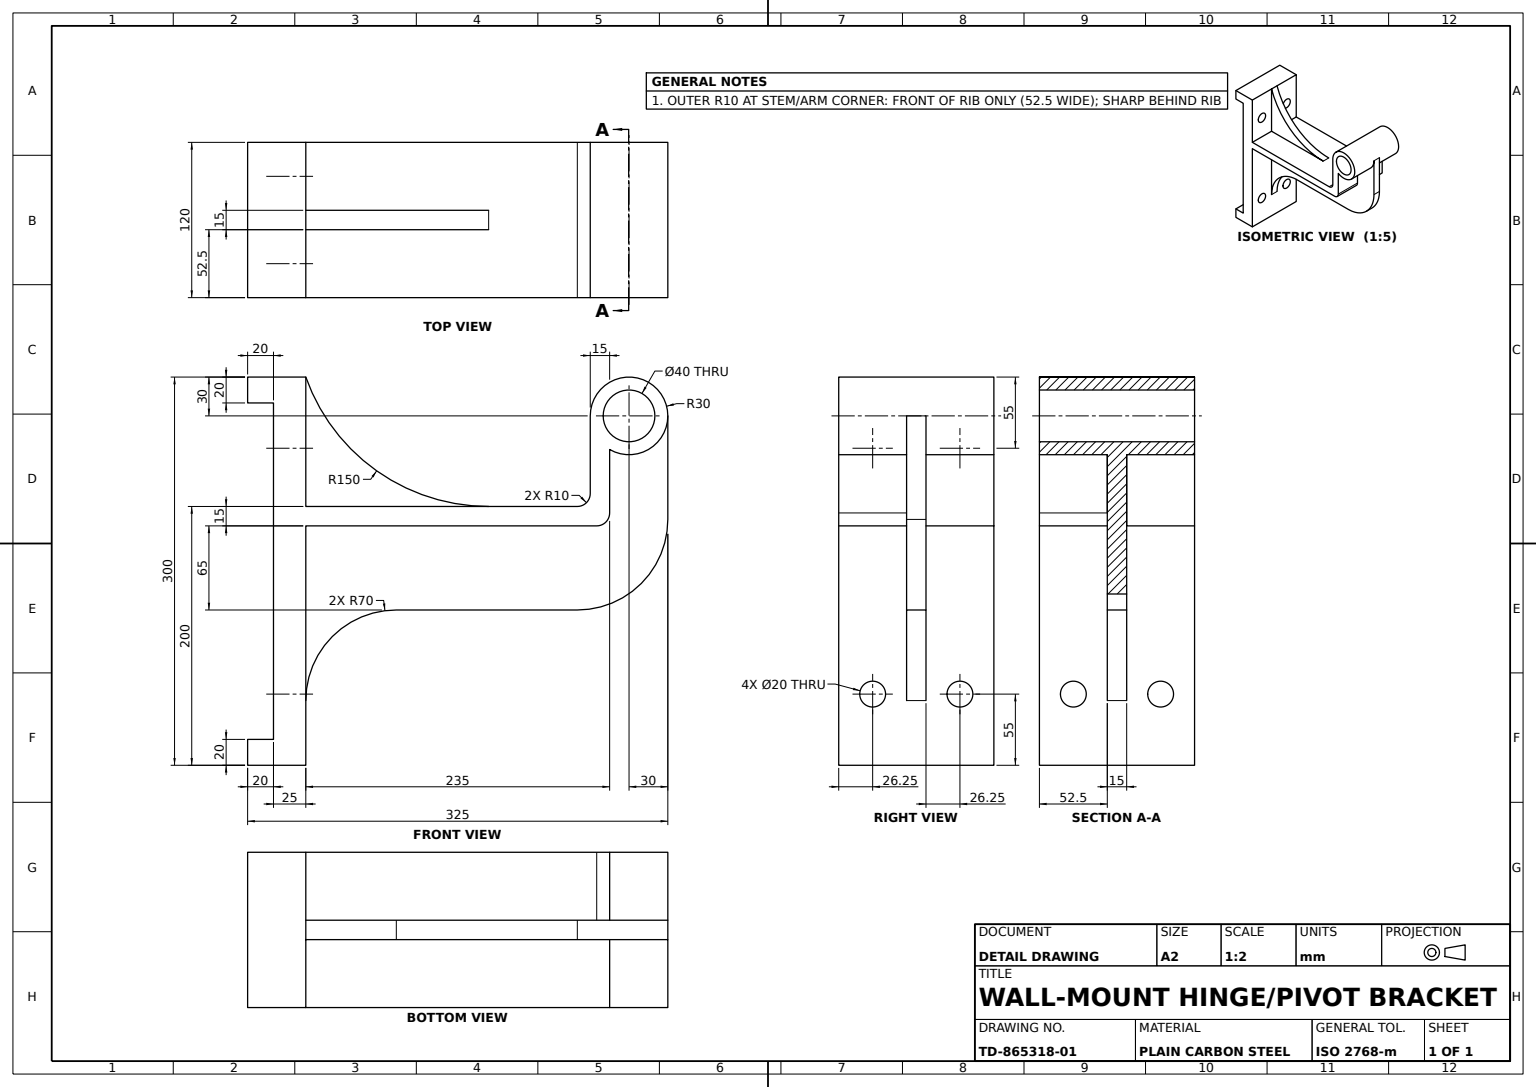
ISO-10303-21;
HEADER;
FILE_DESCRIPTION((''),'2;1');
FILE_NAME('','',(''),(''),'','','');
FILE_SCHEMA(('AUTOMOTIVE_DESIGN'));
ENDSEC;
DATA;
#1=APPLICATION_CONTEXT('');
#2=PRODUCT_CONTEXT('',#1,'mechanical');
#3=PRODUCT('','','',(#2));
#4=PRODUCT_DEFINITION_FORMATION('','',#3);
#5=PRODUCT_DEFINITION_CONTEXT('',#1,'design');
#6=PRODUCT_DEFINITION('','',#4,#5);
#7=PRODUCT_DEFINITION_SHAPE('','',#6);
#8=(LENGTH_UNIT()NAMED_UNIT(*)SI_UNIT(.MILLI.,.METRE.));
#9=(NAMED_UNIT(*)PLANE_ANGLE_UNIT()SI_UNIT($,.RADIAN.));
#10=(NAMED_UNIT(*)SI_UNIT($,.STERADIAN.)SOLID_ANGLE_UNIT());
#11=UNCERTAINTY_MEASURE_WITH_UNIT(LENGTH_MEASURE(1.E-05),#8,'distance_accuracy_value','');
#12=(GEOMETRIC_REPRESENTATION_CONTEXT(3)GLOBAL_UNCERTAINTY_ASSIGNED_CONTEXT((#11))GLOBAL_UNIT_ASSIGNED_CONTEXT((#8,#9,#10))REPRESENTATION_CONTEXT('',''));
#13=CARTESIAN_POINT('',(0.,120.,-292.5));
#14=VERTEX_POINT('',#13);
#15=CARTESIAN_POINT('',(0.,120.,-252.5));
#16=VERTEX_POINT('',#15);
#17=CARTESIAN_POINT('',(0.,120.,-272.5));
#18=DIRECTION('',(1.,0.,0.));
#19=DIRECTION('',(0.,0.,-1.));
#20=AXIS2_PLACEMENT_3D('',#17,#18,#19);
#21=CIRCLE('',#20,20.);
#22=EDGE_CURVE('',#14,#16,#21,.T.);
#23=ORIENTED_EDGE('',*,*,#22,.T.);
#24=CARTESIAN_POINT('',(-120.,120.,-252.5));
#25=VERTEX_POINT('',#24);
#26=VECTOR('',#18,1000.);
#27=LINE('',#24,#26);
#28=EDGE_CURVE('',#25,#16,#27,.T.);
#29=ORIENTED_EDGE('',*,*,#28,.F.);
#30=CARTESIAN_POINT('',(-120.,120.,-292.5));
#31=VERTEX_POINT('',#30);
#32=CARTESIAN_POINT('',(-120.,120.,-272.5));
#33=AXIS2_PLACEMENT_3D('',#32,#18,#19);
#34=CIRCLE('',#33,20.);
#35=EDGE_CURVE('',#31,#25,#34,.T.);
#36=ORIENTED_EDGE('',*,*,#35,.F.);
#37=LINE('',#30,#26);
#38=EDGE_CURVE('',#31,#14,#37,.T.);
#39=ORIENTED_EDGE('',*,*,#38,.T.);
#40=EDGE_LOOP('',(#23,#29,#36,#39));
#41=FACE_OUTER_BOUND('',#40,.T.);
#42=CYLINDRICAL_SURFACE('',#33,20.);
#43=ADVANCED_FACE('',(#41),#42,.F.);
#44=ORIENTED_EDGE('',*,*,#22,.F.);
#45=EDGE_CURVE('',#16,#14,#21,.T.);
#46=ORIENTED_EDGE('',*,*,#45,.F.);
#47=EDGE_LOOP('',(#44,#46));
#48=FACE_BOUND('',#47,.T.);
#49=CARTESIAN_POINT('',(0.,130.,22.5));
#50=VERTEX_POINT('',#49);
#51=CARTESIAN_POINT('',(0.,130.,2.5));
#52=VERTEX_POINT('',#51);
#53=VECTOR('',#19,1000.);
#54=LINE('',#49,#53);
#55=EDGE_CURVE('',#50,#52,#54,.T.);
#56=ORIENTED_EDGE('',*,*,#55,.T.);
#57=CARTESIAN_POINT('',(0.,-130.,2.5));
#58=VERTEX_POINT('',#57);
#59=DIRECTION('',(0.,-1.,0.));
#60=VECTOR('',#59,1000.);
#61=LINE('',#51,#60);
#62=EDGE_CURVE('',#52,#58,#61,.T.);
#63=ORIENTED_EDGE('',*,*,#62,.T.);
#64=CARTESIAN_POINT('',(0.,-130.,22.5));
#65=VERTEX_POINT('',#64);
#66=DIRECTION('',(0.,0.,1.));
#67=VECTOR('',#66,1000.);
#68=LINE('',#57,#67);
#69=EDGE_CURVE('',#58,#65,#68,.T.);
#70=ORIENTED_EDGE('',*,*,#69,.T.);
#71=CARTESIAN_POINT('',(0.,-150.,22.5));
#72=VERTEX_POINT('',#71);
#73=LINE('',#71,#60);
#74=EDGE_CURVE('',#65,#72,#73,.T.);
#75=ORIENTED_EDGE('',*,*,#74,.T.);
#76=CARTESIAN_POINT('',(0.,-150.,-22.5));
#77=VERTEX_POINT('',#76);
#78=LINE('',#71,#53);
#79=EDGE_CURVE('',#72,#77,#78,.T.);
#80=ORIENTED_EDGE('',*,*,#79,.T.);
#81=CARTESIAN_POINT('',(0.,35.,-22.5));
#82=VERTEX_POINT('',#81);
#83=DIRECTION('',(0.,1.,0.));
#84=VECTOR('',#83,1000.);
#85=LINE('',#76,#84);
#86=EDGE_CURVE('',#77,#82,#85,.T.);
#87=ORIENTED_EDGE('',*,*,#86,.T.);
#88=CARTESIAN_POINT('',(0.,35.,-247.5));
#89=VERTEX_POINT('',#88);
#90=CARTESIAN_POINT('',(0.,35.,-257.5));
#91=LINE('',#90,#67);
#92=EDGE_CURVE('',#89,#82,#91,.T.);
#93=ORIENTED_EDGE('',*,*,#92,.F.);
#94=CARTESIAN_POINT('',(0.,45.,-257.5));
#95=VERTEX_POINT('',#94);
#96=CARTESIAN_POINT('',(0.,45.,-247.5));
#97=AXIS2_PLACEMENT_3D('',#96,#18,#66);
#98=CIRCLE('',#97,10.);
#99=EDGE_CURVE('',#89,#95,#98,.T.);
#100=ORIENTED_EDGE('',*,*,#99,.T.);
#101=CARTESIAN_POINT('',(0.,94.019238,-257.5));
#102=VERTEX_POINT('',#101);
#103=CARTESIAN_POINT('',(0.,50.,-257.5));
#104=LINE('',#103,#60);
#105=EDGE_CURVE('',#102,#95,#104,.T.);
#106=ORIENTED_EDGE('',*,*,#105,.F.);
#107=CARTESIAN_POINT('',(0.,120.,-302.5));
#108=VERTEX_POINT('',#107);
#109=CIRCLE('',#20,30.);
#110=EDGE_CURVE('',#102,#108,#109,.T.);
#111=ORIENTED_EDGE('',*,*,#110,.T.);
#112=CARTESIAN_POINT('',(0.,120.,-242.5));
#113=VERTEX_POINT('',#112);
#114=EDGE_CURVE('',#108,#113,#109,.T.);
#115=ORIENTED_EDGE('',*,*,#114,.T.);
#116=CARTESIAN_POINT('',(0.,60.,-242.5));
#117=VERTEX_POINT('',#116);
#118=LINE('',#112,#60);
#119=EDGE_CURVE('',#113,#117,#118,.T.);
#120=ORIENTED_EDGE('',*,*,#119,.T.);
#121=CARTESIAN_POINT('',(0.,50.,-232.5));
#122=VERTEX_POINT('',#121);
#123=CARTESIAN_POINT('',(0.,60.,-232.5));
#124=DIRECTION('',(-1.,0.,0.));
#125=AXIS2_PLACEMENT_3D('',#123,#124,#66);
#126=CIRCLE('',#125,10.);
#127=EDGE_CURVE('',#117,#122,#126,.T.);
#128=ORIENTED_EDGE('',*,*,#127,.T.);
#129=CARTESIAN_POINT('',(0.,50.,-22.5));
#130=VERTEX_POINT('',#129);
#131=LINE('',#103,#67);
#132=EDGE_CURVE('',#122,#130,#131,.T.);
#133=ORIENTED_EDGE('',*,*,#132,.T.);
#134=CARTESIAN_POINT('',(0.,150.,-22.5));
#135=VERTEX_POINT('',#134);
#136=EDGE_CURVE('',#130,#135,#85,.T.);
#137=ORIENTED_EDGE('',*,*,#136,.T.);
#138=CARTESIAN_POINT('',(0.,150.,22.5));
#139=VERTEX_POINT('',#138);
#140=LINE('',#138,#67);
#141=EDGE_CURVE('',#135,#139,#140,.T.);
#142=ORIENTED_EDGE('',*,*,#141,.T.);
#143=LINE('',#49,#60);
#144=EDGE_CURVE('',#139,#50,#143,.T.);
#145=ORIENTED_EDGE('',*,*,#144,.T.);
#146=EDGE_LOOP('',(#56,#63,#70,#75,#80,#87,#93,#100,#106,#111,#115,#120,#128,#133,#137,#142,#145));
#147=FACE_OUTER_BOUND('',#146,.T.);
#148=CARTESIAN_POINT('',(0.,0.,0.));
#149=AXIS2_PLACEMENT_3D('',#148,#124,#66);
#150=PLANE('',#149);
#151=ADVANCED_FACE('',(#48,#147),#150,.F.);
#152=CARTESIAN_POINT('',(-67.5,150.,-22.5));
#153=VERTEX_POINT('',#152);
#154=CARTESIAN_POINT('',(-52.5,150.,-22.5));
#155=VERTEX_POINT('',#154);
#156=CARTESIAN_POINT('',(-60.,150.,-22.5));
#157=LINE('',#156,#26);
#158=EDGE_CURVE('',#153,#155,#157,.T.);
#159=ORIENTED_EDGE('',*,*,#158,.F.);
#160=CARTESIAN_POINT('',(-120.,150.,-22.5));
#161=VERTEX_POINT('',#160);
#162=LINE('',#160,#26);
#163=EDGE_CURVE('',#161,#153,#162,.T.);
#164=ORIENTED_EDGE('',*,*,#163,.F.);
#165=CARTESIAN_POINT('',(-120.,150.,22.5));
#166=VERTEX_POINT('',#165);
#167=LINE('',#165,#67);
#168=EDGE_CURVE('',#161,#166,#167,.T.);
#169=ORIENTED_EDGE('',*,*,#168,.T.);
#170=LINE('',#165,#26);
#171=EDGE_CURVE('',#166,#139,#170,.T.);
#172=ORIENTED_EDGE('',*,*,#171,.T.);
#173=ORIENTED_EDGE('',*,*,#141,.F.);
#174=EDGE_CURVE('',#155,#135,#162,.T.);
#175=ORIENTED_EDGE('',*,*,#174,.F.);
#176=EDGE_LOOP('',(#159,#164,#169,#172,#173,#175));
#177=FACE_OUTER_BOUND('',#176,.T.);
#178=AXIS2_PLACEMENT_3D('',#165,#83,#66);
#179=PLANE('',#178);
#180=ADVANCED_FACE('',(#177),#179,.T.);
#181=CARTESIAN_POINT('',(-67.5,-30.,-92.5));
#182=VERTEX_POINT('',#181);
#183=CARTESIAN_POINT('',(-67.5,-30.,-232.5));
#184=VERTEX_POINT('',#183);
#185=LINE('',#181,#53);
#186=EDGE_CURVE('',#182,#184,#185,.T.);
#187=ORIENTED_EDGE('',*,*,#186,.F.);
#188=CARTESIAN_POINT('',(-67.5,-100.,-22.5));
#189=VERTEX_POINT('',#188);
#190=CARTESIAN_POINT('',(-67.5,-100.,-92.5));
#191=AXIS2_PLACEMENT_3D('',#190,#124,#66);
#192=CIRCLE('',#191,70.);
#193=EDGE_CURVE('',#189,#182,#192,.T.);
#194=ORIENTED_EDGE('',*,*,#193,.F.);
#195=CARTESIAN_POINT('',(-67.5,35.,-22.5));
#196=VERTEX_POINT('',#195);
#197=LINE('',#188,#60);
#198=EDGE_CURVE('',#196,#189,#197,.T.);
#199=ORIENTED_EDGE('',*,*,#198,.F.);
#200=CARTESIAN_POINT('',(-67.5,35.,-257.5));
#201=VERTEX_POINT('',#200);
#202=LINE('',#195,#67);
#203=EDGE_CURVE('',#201,#196,#202,.T.);
#204=ORIENTED_EDGE('',*,*,#203,.F.);
#205=CARTESIAN_POINT('',(-67.5,94.019238,-257.5));
#206=VERTEX_POINT('',#205);
#207=LINE('',#200,#60);
#208=EDGE_CURVE('',#206,#201,#207,.T.);
#209=ORIENTED_EDGE('',*,*,#208,.F.);
#210=CARTESIAN_POINT('',(-67.5,120.,-302.5));
#211=VERTEX_POINT('',#210);
#212=CARTESIAN_POINT('',(-67.5,120.,-272.5));
#213=AXIS2_PLACEMENT_3D('',#212,#124,#19);
#214=CIRCLE('',#213,30.);
#215=EDGE_CURVE('',#211,#206,#214,.T.);
#216=ORIENTED_EDGE('',*,*,#215,.F.);
#217=CARTESIAN_POINT('',(-67.5,40.,-302.5));
#218=VERTEX_POINT('',#217);
#219=LINE('',#210,#84);
#220=EDGE_CURVE('',#218,#211,#219,.T.);
#221=ORIENTED_EDGE('',*,*,#220,.F.);
#222=CARTESIAN_POINT('',(-67.5,40.,-232.5));
#223=AXIS2_PLACEMENT_3D('',#222,#18,#19);
#224=CIRCLE('',#223,70.);
#225=EDGE_CURVE('',#184,#218,#224,.T.);
#226=ORIENTED_EDGE('',*,*,#225,.F.);
#227=EDGE_LOOP('',(#187,#194,#199,#204,#209,#216,#221,#226));
#228=FACE_OUTER_BOUND('',#227,.T.);
#229=AXIS2_PLACEMENT_3D('',#212,#18,#19);
#230=PLANE('',#229);
#231=ADVANCED_FACE('',(#228),#230,.F.);
#232=CARTESIAN_POINT('',(-120.,-130.,2.5));
#233=VERTEX_POINT('',#232);
#234=CARTESIAN_POINT('',(-120.,-130.,22.5));
#235=VERTEX_POINT('',#234);
#236=LINE('',#232,#67);
#237=EDGE_CURVE('',#233,#235,#236,.T.);
#238=ORIENTED_EDGE('',*,*,#237,.T.);
#239=LINE('',#234,#26);
#240=EDGE_CURVE('',#235,#65,#239,.T.);
#241=ORIENTED_EDGE('',*,*,#240,.T.);
#242=ORIENTED_EDGE('',*,*,#69,.F.);
#243=LINE('',#232,#26);
#244=EDGE_CURVE('',#233,#58,#243,.T.);
#245=ORIENTED_EDGE('',*,*,#244,.F.);
#246=EDGE_LOOP('',(#238,#241,#242,#245));
#247=FACE_OUTER_BOUND('',#246,.T.);
#248=AXIS2_PLACEMENT_3D('',#232,#83,#66);
#249=PLANE('',#248);
#250=ADVANCED_FACE('',(#247),#249,.T.);
#251=CARTESIAN_POINT('',(-120.,-150.,22.5));
#252=VERTEX_POINT('',#251);
#253=CARTESIAN_POINT('',(-120.,-150.,-22.5));
#254=VERTEX_POINT('',#253);
#255=LINE('',#251,#53);
#256=EDGE_CURVE('',#252,#254,#255,.T.);
#257=ORIENTED_EDGE('',*,*,#256,.F.);
#258=LINE('',#251,#60);
#259=EDGE_CURVE('',#235,#252,#258,.T.);
#260=ORIENTED_EDGE('',*,*,#259,.F.);
#261=ORIENTED_EDGE('',*,*,#237,.F.);
#262=CARTESIAN_POINT('',(-120.,130.,2.5));
#263=VERTEX_POINT('',#262);
#264=LINE('',#262,#60);
#265=EDGE_CURVE('',#263,#233,#264,.T.);
#266=ORIENTED_EDGE('',*,*,#265,.F.);
#267=CARTESIAN_POINT('',(-120.,130.,22.5));
#268=VERTEX_POINT('',#267);
#269=LINE('',#267,#53);
#270=EDGE_CURVE('',#268,#263,#269,.T.);
#271=ORIENTED_EDGE('',*,*,#270,.F.);
#272=LINE('',#267,#60);
#273=EDGE_CURVE('',#166,#268,#272,.T.);
#274=ORIENTED_EDGE('',*,*,#273,.F.);
#275=ORIENTED_EDGE('',*,*,#168,.F.);
#276=CARTESIAN_POINT('',(-120.,50.,-22.5));
#277=VERTEX_POINT('',#276);
#278=LINE('',#253,#84);
#279=EDGE_CURVE('',#277,#161,#278,.T.);
#280=ORIENTED_EDGE('',*,*,#279,.F.);
#281=CARTESIAN_POINT('',(-120.,50.,-232.5));
#282=VERTEX_POINT('',#281);
#283=CARTESIAN_POINT('',(-120.,50.,-257.5));
#284=LINE('',#283,#67);
#285=EDGE_CURVE('',#282,#277,#284,.T.);
#286=ORIENTED_EDGE('',*,*,#285,.F.);
#287=CARTESIAN_POINT('',(-120.,60.,-242.5));
#288=VERTEX_POINT('',#287);
#289=CARTESIAN_POINT('',(-120.,60.,-232.5));
#290=AXIS2_PLACEMENT_3D('',#289,#18,#66);
#291=CIRCLE('',#290,10.);
#292=EDGE_CURVE('',#282,#288,#291,.T.);
#293=ORIENTED_EDGE('',*,*,#292,.T.);
#294=CARTESIAN_POINT('',(-120.,120.,-242.5));
#295=VERTEX_POINT('',#294);
#296=LINE('',#294,#60);
#297=EDGE_CURVE('',#295,#288,#296,.T.);
#298=ORIENTED_EDGE('',*,*,#297,.F.);
#299=CARTESIAN_POINT('',(-120.,120.,-302.5));
#300=VERTEX_POINT('',#299);
#301=CIRCLE('',#33,30.);
#302=EDGE_CURVE('',#300,#295,#301,.T.);
#303=ORIENTED_EDGE('',*,*,#302,.F.);
#304=CARTESIAN_POINT('',(-120.,94.019238,-257.5));
#305=VERTEX_POINT('',#304);
#306=EDGE_CURVE('',#305,#300,#301,.T.);
#307=ORIENTED_EDGE('',*,*,#306,.F.);
#308=CARTESIAN_POINT('',(-120.,35.,-257.5));
#309=VERTEX_POINT('',#308);
#310=LINE('',#283,#84);
#311=EDGE_CURVE('',#309,#305,#310,.T.);
#312=ORIENTED_EDGE('',*,*,#311,.F.);
#313=CARTESIAN_POINT('',(-120.,35.,-22.5));
#314=VERTEX_POINT('',#313);
#315=LINE('',#308,#67);
#316=EDGE_CURVE('',#309,#314,#315,.T.);
#317=ORIENTED_EDGE('',*,*,#316,.T.);
#318=EDGE_CURVE('',#254,#314,#278,.T.);
#319=ORIENTED_EDGE('',*,*,#318,.F.);
#320=EDGE_LOOP('',(#257,#260,#261,#266,#271,#274,#275,#280,#286,#293,#298,#303,#307,#312,#317,#319));
#321=FACE_OUTER_BOUND('',#320,.T.);
#322=ORIENTED_EDGE('',*,*,#35,.T.);
#323=EDGE_CURVE('',#25,#31,#34,.T.);
#324=ORIENTED_EDGE('',*,*,#323,.T.);
#325=EDGE_LOOP('',(#322,#324));
#326=FACE_BOUND('',#325,.T.);
#327=CARTESIAN_POINT('',(-120.,0.,0.));
#328=AXIS2_PLACEMENT_3D('',#327,#124,#66);
#329=PLANE('',#328);
#330=ADVANCED_FACE('',(#321,#326),#329,.T.);
#331=CARTESIAN_POINT('',(-103.75,95.,2.5));
#332=VERTEX_POINT('',#331);
#333=CARTESIAN_POINT('',(-103.75,95.,-22.5));
#334=VERTEX_POINT('',#333);
#335=CARTESIAN_POINT('',(-103.75,95.,22.5));
#336=LINE('',#335,#53);
#337=EDGE_CURVE('',#332,#334,#336,.T.);
#338=ORIENTED_EDGE('',*,*,#337,.F.);
#339=CARTESIAN_POINT('',(-83.75,95.,2.5));
#340=VERTEX_POINT('',#339);
#341=CARTESIAN_POINT('',(-93.75,95.,2.5));
#342=AXIS2_PLACEMENT_3D('',#341,#66,#59);
#343=CIRCLE('',#342,10.);
#344=EDGE_CURVE('',#332,#340,#343,.T.);
#345=ORIENTED_EDGE('',*,*,#344,.T.);
#346=CARTESIAN_POINT('',(-83.75,95.,-22.5));
#347=VERTEX_POINT('',#346);
#348=CARTESIAN_POINT('',(-83.75,95.,22.5));
#349=LINE('',#348,#53);
#350=EDGE_CURVE('',#340,#347,#349,.T.);
#351=ORIENTED_EDGE('',*,*,#350,.T.);
#352=CARTESIAN_POINT('',(-93.75,95.,-22.5));
#353=AXIS2_PLACEMENT_3D('',#352,#19,#124);
#354=CIRCLE('',#353,10.);
#355=EDGE_CURVE('',#347,#334,#354,.T.);
#356=ORIENTED_EDGE('',*,*,#355,.T.);
#357=EDGE_LOOP('',(#338,#345,#351,#356));
#358=FACE_OUTER_BOUND('',#357,.T.);
#359=CARTESIAN_POINT('',(-93.75,95.,22.5));
#360=AXIS2_PLACEMENT_3D('',#359,#19,#124);
#361=CYLINDRICAL_SURFACE('',#360,10.);
#362=ADVANCED_FACE('',(#358),#361,.F.);
#363=CARTESIAN_POINT('',(-52.5,50.,-163.921356));
#364=VERTEX_POINT('',#363);
#365=CARTESIAN_POINT('',(-52.5,200.,-163.921356));
#366=AXIS2_PLACEMENT_3D('',#365,#18,#19);
#367=CIRCLE('',#366,150.);
#368=EDGE_CURVE('',#155,#364,#367,.T.);
#369=ORIENTED_EDGE('',*,*,#368,.T.);
#370=CARTESIAN_POINT('',(-67.5,50.,-163.921356));
#371=VERTEX_POINT('',#370);
#372=CARTESIAN_POINT('',(-60.,50.,-163.921356));
#373=LINE('',#372,#26);
#374=EDGE_CURVE('',#371,#364,#373,.T.);
#375=ORIENTED_EDGE('',*,*,#374,.F.);
#376=CARTESIAN_POINT('',(-67.5,200.,-163.921356));
#377=AXIS2_PLACEMENT_3D('',#376,#18,#19);
#378=CIRCLE('',#377,150.);
#379=EDGE_CURVE('',#153,#371,#378,.T.);
#380=ORIENTED_EDGE('',*,*,#379,.F.);
#381=ORIENTED_EDGE('',*,*,#158,.T.);
#382=EDGE_LOOP('',(#369,#375,#380,#381));
#383=FACE_OUTER_BOUND('',#382,.T.);
#384=CARTESIAN_POINT('',(-60.,200.,-163.921356));
#385=AXIS2_PLACEMENT_3D('',#384,#18,#19);
#386=CYLINDRICAL_SURFACE('',#385,150.);
#387=ADVANCED_FACE('',(#383),#386,.F.);
#388=CARTESIAN_POINT('',(-36.25,95.,2.5));
#389=VERTEX_POINT('',#388);
#390=CARTESIAN_POINT('',(-16.25,95.,2.5));
#391=VERTEX_POINT('',#390);
#392=CARTESIAN_POINT('',(-26.25,95.,2.5));
#393=AXIS2_PLACEMENT_3D('',#392,#66,#59);
#394=CIRCLE('',#393,10.);
#395=EDGE_CURVE('',#389,#391,#394,.T.);
#396=ORIENTED_EDGE('',*,*,#395,.T.);
#397=CARTESIAN_POINT('',(-16.25,95.,-22.5));
#398=VERTEX_POINT('',#397);
#399=CARTESIAN_POINT('',(-16.25,95.,22.5));
#400=LINE('',#399,#53);
#401=EDGE_CURVE('',#391,#398,#400,.T.);
#402=ORIENTED_EDGE('',*,*,#401,.T.);
#403=CARTESIAN_POINT('',(-36.25,95.,-22.5));
#404=VERTEX_POINT('',#403);
#405=CARTESIAN_POINT('',(-26.25,95.,-22.5));
#406=AXIS2_PLACEMENT_3D('',#405,#19,#124);
#407=CIRCLE('',#406,10.);
#408=EDGE_CURVE('',#398,#404,#407,.T.);
#409=ORIENTED_EDGE('',*,*,#408,.T.);
#410=CARTESIAN_POINT('',(-36.25,95.,22.5));
#411=LINE('',#410,#53);
#412=EDGE_CURVE('',#389,#404,#411,.T.);
#413=ORIENTED_EDGE('',*,*,#412,.F.);
#414=EDGE_LOOP('',(#396,#402,#409,#413));
#415=FACE_OUTER_BOUND('',#414,.T.);
#416=CARTESIAN_POINT('',(-26.25,95.,22.5));
#417=AXIS2_PLACEMENT_3D('',#416,#19,#124);
#418=CYLINDRICAL_SURFACE('',#417,10.);
#419=ADVANCED_FACE('',(#415),#418,.F.);
#420=CARTESIAN_POINT('',(-52.5,50.,-22.5));
#421=VERTEX_POINT('',#420);
#422=CARTESIAN_POINT('',(-52.5,50.,-257.5));
#423=LINE('',#422,#67);
#424=EDGE_CURVE('',#364,#421,#423,.T.);
#425=ORIENTED_EDGE('',*,*,#424,.F.);
#426=ORIENTED_EDGE('',*,*,#368,.F.);
#427=CARTESIAN_POINT('',(-52.5,-150.,-22.5));
#428=LINE('',#427,#60);
#429=EDGE_CURVE('',#155,#421,#428,.T.);
#430=ORIENTED_EDGE('',*,*,#429,.T.);
#431=EDGE_LOOP('',(#425,#426,#430));
#432=FACE_OUTER_BOUND('',#431,.T.);
#433=CARTESIAN_POINT('',(-52.5,0.,-140.));
#434=AXIS2_PLACEMENT_3D('',#433,#18,#19);
#435=PLANE('',#434);
#436=ADVANCED_FACE('',(#432),#435,.T.);
#437=ORIENTED_EDGE('',*,*,#429,.F.);
#438=ORIENTED_EDGE('',*,*,#174,.T.);
#439=ORIENTED_EDGE('',*,*,#136,.F.);
#440=LINE('',#129,#26);
#441=EDGE_CURVE('',#421,#130,#440,.T.);
#442=ORIENTED_EDGE('',*,*,#441,.F.);
#443=EDGE_LOOP('',(#437,#438,#439,#442));
#444=FACE_OUTER_BOUND('',#443,.T.);
#445=ORIENTED_EDGE('',*,*,#408,.F.);
#446=EDGE_CURVE('',#404,#398,#407,.T.);
#447=ORIENTED_EDGE('',*,*,#446,.F.);
#448=EDGE_LOOP('',(#445,#447));
#449=FACE_BOUND('',#448,.T.);
#450=AXIS2_PLACEMENT_3D('',#253,#19,#124);
#451=PLANE('',#450);
#452=ADVANCED_FACE('',(#444,#449),#451,.T.);
#453=ORIENTED_EDGE('',*,*,#401,.F.);
#454=EDGE_CURVE('',#391,#389,#394,.T.);
#455=ORIENTED_EDGE('',*,*,#454,.T.);
#456=ORIENTED_EDGE('',*,*,#412,.T.);
#457=ORIENTED_EDGE('',*,*,#446,.T.);
#458=EDGE_LOOP('',(#453,#455,#456,#457));
#459=FACE_OUTER_BOUND('',#458,.T.);
#460=ADVANCED_FACE('',(#459),#418,.F.);
#461=CARTESIAN_POINT('',(-16.25,-95.,2.5));
#462=VERTEX_POINT('',#461);
#463=CARTESIAN_POINT('',(-16.25,-95.,-22.5));
#464=VERTEX_POINT('',#463);
#465=CARTESIAN_POINT('',(-16.25,-95.,22.5));
#466=LINE('',#465,#53);
#467=EDGE_CURVE('',#462,#464,#466,.T.);
#468=ORIENTED_EDGE('',*,*,#467,.T.);
#469=CARTESIAN_POINT('',(-36.25,-95.,-22.5));
#470=VERTEX_POINT('',#469);
#471=CARTESIAN_POINT('',(-26.25,-95.,-22.5));
#472=AXIS2_PLACEMENT_3D('',#471,#19,#124);
#473=CIRCLE('',#472,10.);
#474=EDGE_CURVE('',#464,#470,#473,.T.);
#475=ORIENTED_EDGE('',*,*,#474,.T.);
#476=CARTESIAN_POINT('',(-36.25,-95.,2.5));
#477=VERTEX_POINT('',#476);
#478=CARTESIAN_POINT('',(-36.25,-95.,22.5));
#479=LINE('',#478,#53);
#480=EDGE_CURVE('',#477,#470,#479,.T.);
#481=ORIENTED_EDGE('',*,*,#480,.F.);
#482=CARTESIAN_POINT('',(-26.25,-95.,2.5));
#483=AXIS2_PLACEMENT_3D('',#482,#66,#59);
#484=CIRCLE('',#483,10.);
#485=EDGE_CURVE('',#477,#462,#484,.T.);
#486=ORIENTED_EDGE('',*,*,#485,.T.);
#487=EDGE_LOOP('',(#468,#475,#481,#486));
#488=FACE_OUTER_BOUND('',#487,.T.);
#489=CARTESIAN_POINT('',(-26.25,-95.,22.5));
#490=AXIS2_PLACEMENT_3D('',#489,#19,#124);
#491=CYLINDRICAL_SURFACE('',#490,10.);
#492=ADVANCED_FACE('',(#488),#491,.F.);
#493=VECTOR('',#124,1000.);
#494=LINE('',#81,#493);
#495=EDGE_CURVE('',#196,#314,#494,.T.);
#496=ORIENTED_EDGE('',*,*,#495,.T.);
#497=ORIENTED_EDGE('',*,*,#316,.F.);
#498=LINE('',#90,#493);
#499=EDGE_CURVE('',#201,#309,#498,.T.);
#500=ORIENTED_EDGE('',*,*,#499,.F.);
#501=ORIENTED_EDGE('',*,*,#203,.T.);
#502=EDGE_LOOP('',(#496,#497,#500,#501));
#503=FACE_OUTER_BOUND('',#502,.T.);
#504=AXIS2_PLACEMENT_3D('',#90,#83,#66);
#505=PLANE('',#504);
#506=ADVANCED_FACE('',(#503),#505,.F.);
#507=ORIENTED_EDGE('',*,*,#467,.F.);
#508=EDGE_CURVE('',#462,#477,#484,.T.);
#509=ORIENTED_EDGE('',*,*,#508,.T.);
#510=ORIENTED_EDGE('',*,*,#480,.T.);
#511=EDGE_CURVE('',#470,#464,#473,.T.);
#512=ORIENTED_EDGE('',*,*,#511,.T.);
#513=EDGE_LOOP('',(#507,#509,#510,#512));
#514=FACE_OUTER_BOUND('',#513,.T.);
#515=ADVANCED_FACE('',(#514),#491,.F.);
#516=CARTESIAN_POINT('',(-52.5,40.,-302.5));
#517=VERTEX_POINT('',#516);
#518=LINE('',#516,#493);
#519=EDGE_CURVE('',#517,#218,#518,.T.);
#520=ORIENTED_EDGE('',*,*,#519,.T.);
#521=ORIENTED_EDGE('',*,*,#220,.T.);
#522=CARTESIAN_POINT('',(-52.5,120.,-302.5));
#523=VERTEX_POINT('',#522);
#524=LINE('',#522,#493);
#525=EDGE_CURVE('',#523,#211,#524,.T.);
#526=ORIENTED_EDGE('',*,*,#525,.F.);
#527=LINE('',#522,#84);
#528=EDGE_CURVE('',#517,#523,#527,.T.);
#529=ORIENTED_EDGE('',*,*,#528,.F.);
#530=EDGE_LOOP('',(#520,#521,#526,#529));
#531=FACE_OUTER_BOUND('',#530,.T.);
#532=AXIS2_PLACEMENT_3D('',#522,#66,#59);
#533=PLANE('',#532);
#534=ADVANCED_FACE('',(#531),#533,.F.);
#535=LINE('',#304,#26);
#536=EDGE_CURVE('',#305,#206,#535,.T.);
#537=ORIENTED_EDGE('',*,*,#536,.F.);
#538=ORIENTED_EDGE('',*,*,#306,.T.);
#539=LINE('',#299,#26);
#540=EDGE_CURVE('',#300,#211,#539,.T.);
#541=ORIENTED_EDGE('',*,*,#540,.T.);
#542=ORIENTED_EDGE('',*,*,#215,.T.);
#543=EDGE_LOOP('',(#537,#538,#541,#542));
#544=FACE_OUTER_BOUND('',#543,.T.);
#545=CYLINDRICAL_SURFACE('',#33,30.);
#546=ADVANCED_FACE('',(#544),#545,.T.);
#547=CARTESIAN_POINT('',(-52.5,35.,-22.5));
#548=VERTEX_POINT('',#547);
#549=EDGE_CURVE('',#82,#548,#494,.T.);
#550=ORIENTED_EDGE('',*,*,#549,.T.);
#551=CARTESIAN_POINT('',(-52.5,35.,-247.5));
#552=VERTEX_POINT('',#551);
#553=LINE('',#547,#67);
#554=EDGE_CURVE('',#552,#548,#553,.T.);
#555=ORIENTED_EDGE('',*,*,#554,.F.);
#556=LINE('',#88,#26);
#557=EDGE_CURVE('',#552,#89,#556,.T.);
#558=ORIENTED_EDGE('',*,*,#557,.T.);
#559=ORIENTED_EDGE('',*,*,#92,.T.);
#560=EDGE_LOOP('',(#550,#555,#558,#559));
#561=FACE_OUTER_BOUND('',#560,.T.);
#562=ADVANCED_FACE('',(#561),#505,.F.);
#563=LINE('',#267,#26);
#564=EDGE_CURVE('',#268,#50,#563,.T.);
#565=ORIENTED_EDGE('',*,*,#564,.T.);
#566=ORIENTED_EDGE('',*,*,#144,.F.);
#567=ORIENTED_EDGE('',*,*,#171,.F.);
#568=ORIENTED_EDGE('',*,*,#273,.T.);
#569=EDGE_LOOP('',(#565,#566,#567,#568));
#570=FACE_OUTER_BOUND('',#569,.T.);
#571=AXIS2_PLACEMENT_3D('',#267,#66,#18);
#572=PLANE('',#571);
#573=ADVANCED_FACE('',(#570),#572,.T.);
#574=LINE('',#294,#26);
#575=EDGE_CURVE('',#295,#113,#574,.T.);
#576=ORIENTED_EDGE('',*,*,#575,.F.);
#577=ORIENTED_EDGE('',*,*,#297,.T.);
#578=LINE('',#287,#26);
#579=EDGE_CURVE('',#288,#117,#578,.T.);
#580=ORIENTED_EDGE('',*,*,#579,.T.);
#581=ORIENTED_EDGE('',*,*,#119,.F.);
#582=EDGE_LOOP('',(#576,#577,#580,#581));
#583=FACE_OUTER_BOUND('',#582,.T.);
#584=AXIS2_PLACEMENT_3D('',#294,#66,#18);
#585=PLANE('',#584);
#586=ADVANCED_FACE('',(#583),#585,.T.);
#587=LINE('',#262,#26);
#588=EDGE_CURVE('',#263,#52,#587,.T.);
#589=ORIENTED_EDGE('',*,*,#588,.T.);
#590=ORIENTED_EDGE('',*,*,#55,.F.);
#591=ORIENTED_EDGE('',*,*,#564,.F.);
#592=ORIENTED_EDGE('',*,*,#270,.T.);
#593=EDGE_LOOP('',(#589,#590,#591,#592));
#594=FACE_OUTER_BOUND('',#593,.T.);
#595=AXIS2_PLACEMENT_3D('',#267,#59,#19);
#596=PLANE('',#595);
#597=ADVANCED_FACE('',(#594),#596,.T.);
#598=LINE('',#251,#26);
#599=EDGE_CURVE('',#252,#72,#598,.T.);
#600=ORIENTED_EDGE('',*,*,#599,.T.);
#601=ORIENTED_EDGE('',*,*,#74,.F.);
#602=ORIENTED_EDGE('',*,*,#240,.F.);
#603=ORIENTED_EDGE('',*,*,#259,.T.);
#604=EDGE_LOOP('',(#600,#601,#602,#603));
#605=FACE_OUTER_BOUND('',#604,.T.);
#606=AXIS2_PLACEMENT_3D('',#251,#66,#18);
#607=PLANE('',#606);
#608=ADVANCED_FACE('',(#605),#607,.T.);
#609=ORIENTED_EDGE('',*,*,#99,.F.);
#610=ORIENTED_EDGE('',*,*,#557,.F.);
#611=CARTESIAN_POINT('',(-52.5,45.,-257.5));
#612=VERTEX_POINT('',#611);
#613=CARTESIAN_POINT('',(-52.5,45.,-247.5));
#614=AXIS2_PLACEMENT_3D('',#613,#124,#19);
#615=CIRCLE('',#614,10.);
#616=EDGE_CURVE('',#612,#552,#615,.T.);
#617=ORIENTED_EDGE('',*,*,#616,.F.);
#618=LINE('',#611,#493);
#619=EDGE_CURVE('',#95,#612,#618,.T.);
#620=ORIENTED_EDGE('',*,*,#619,.F.);
#621=EDGE_LOOP('',(#609,#610,#617,#620));
#622=FACE_OUTER_BOUND('',#621,.T.);
#623=AXIS2_PLACEMENT_3D('',#96,#18,#19);
#624=CYLINDRICAL_SURFACE('',#623,10.);
#625=ADVANCED_FACE('',(#622),#624,.T.);
#626=ORIENTED_EDGE('',*,*,#186,.T.);
#627=CARTESIAN_POINT('',(-52.5,-30.,-232.5));
#628=VERTEX_POINT('',#627);
#629=LINE('',#627,#493);
#630=EDGE_CURVE('',#628,#184,#629,.T.);
#631=ORIENTED_EDGE('',*,*,#630,.F.);
#632=CARTESIAN_POINT('',(-52.5,-30.,-92.5));
#633=VERTEX_POINT('',#632);
#634=LINE('',#632,#53);
#635=EDGE_CURVE('',#633,#628,#634,.T.);
#636=ORIENTED_EDGE('',*,*,#635,.F.);
#637=LINE('',#632,#493);
#638=EDGE_CURVE('',#633,#182,#637,.T.);
#639=ORIENTED_EDGE('',*,*,#638,.T.);
#640=EDGE_LOOP('',(#626,#631,#636,#639));
#641=FACE_OUTER_BOUND('',#640,.T.);
#642=AXIS2_PLACEMENT_3D('',#632,#83,#66);
#643=PLANE('',#642);
#644=ADVANCED_FACE('',(#641),#643,.F.);
#645=CARTESIAN_POINT('',(-103.75,-95.,2.5));
#646=VERTEX_POINT('',#645);
#647=CARTESIAN_POINT('',(-83.75,-95.,2.5));
#648=VERTEX_POINT('',#647);
#649=CARTESIAN_POINT('',(-93.75,-95.,2.5));
#650=AXIS2_PLACEMENT_3D('',#649,#66,#59);
#651=CIRCLE('',#650,10.);
#652=EDGE_CURVE('',#646,#648,#651,.T.);
#653=ORIENTED_EDGE('',*,*,#652,.F.);
#654=EDGE_CURVE('',#648,#646,#651,.T.);
#655=ORIENTED_EDGE('',*,*,#654,.F.);
#656=EDGE_LOOP('',(#653,#655));
#657=FACE_BOUND('',#656,.T.);
#658=ORIENTED_EDGE('',*,*,#508,.F.);
#659=ORIENTED_EDGE('',*,*,#485,.F.);
#660=EDGE_LOOP('',(#658,#659));
#661=FACE_BOUND('',#660,.T.);
#662=ORIENTED_EDGE('',*,*,#395,.F.);
#663=ORIENTED_EDGE('',*,*,#454,.F.);
#664=EDGE_LOOP('',(#662,#663));
#665=FACE_BOUND('',#664,.T.);
#666=ORIENTED_EDGE('',*,*,#588,.F.);
#667=ORIENTED_EDGE('',*,*,#265,.T.);
#668=ORIENTED_EDGE('',*,*,#244,.T.);
#669=ORIENTED_EDGE('',*,*,#62,.F.);
#670=EDGE_LOOP('',(#666,#667,#668,#669));
#671=FACE_OUTER_BOUND('',#670,.T.);
#672=EDGE_CURVE('',#340,#332,#343,.T.);
#673=ORIENTED_EDGE('',*,*,#672,.F.);
#674=ORIENTED_EDGE('',*,*,#344,.F.);
#675=EDGE_LOOP('',(#673,#674));
#676=FACE_BOUND('',#675,.T.);
#677=AXIS2_PLACEMENT_3D('',#262,#66,#59);
#678=PLANE('',#677);
#679=ADVANCED_FACE('',(#657,#661,#665,#671,#676),#678,.T.);
#680=CARTESIAN_POINT('',(-52.5,-100.,-22.5));
#681=VERTEX_POINT('',#680);
#682=LINE('',#680,#493);
#683=EDGE_CURVE('',#681,#189,#682,.T.);
#684=ORIENTED_EDGE('',*,*,#683,.T.);
#685=ORIENTED_EDGE('',*,*,#193,.T.);
#686=ORIENTED_EDGE('',*,*,#638,.F.);
#687=CARTESIAN_POINT('',(-52.5,-100.,-92.5));
#688=AXIS2_PLACEMENT_3D('',#687,#124,#66);
#689=CIRCLE('',#688,70.);
#690=EDGE_CURVE('',#681,#633,#689,.T.);
#691=ORIENTED_EDGE('',*,*,#690,.F.);
#692=EDGE_LOOP('',(#684,#685,#686,#691));
#693=FACE_OUTER_BOUND('',#692,.T.);
#694=CYLINDRICAL_SURFACE('',#688,70.);
#695=ADVANCED_FACE('',(#693),#694,.F.);
#696=ORIENTED_EDGE('',*,*,#683,.F.);
#697=LINE('',#680,#60);
#698=EDGE_CURVE('',#548,#681,#697,.T.);
#699=ORIENTED_EDGE('',*,*,#698,.F.);
#700=ORIENTED_EDGE('',*,*,#549,.F.);
#701=ORIENTED_EDGE('',*,*,#86,.F.);
#702=LINE('',#253,#26);
#703=EDGE_CURVE('',#254,#77,#702,.T.);
#704=ORIENTED_EDGE('',*,*,#703,.F.);
#705=ORIENTED_EDGE('',*,*,#318,.T.);
#706=ORIENTED_EDGE('',*,*,#495,.F.);
#707=ORIENTED_EDGE('',*,*,#198,.T.);
#708=EDGE_LOOP('',(#696,#699,#700,#701,#704,#705,#706,#707));
#709=FACE_OUTER_BOUND('',#708,.T.);
#710=ORIENTED_EDGE('',*,*,#474,.F.);
#711=ORIENTED_EDGE('',*,*,#511,.F.);
#712=EDGE_LOOP('',(#710,#711));
#713=FACE_BOUND('',#712,.T.);
#714=CARTESIAN_POINT('',(-83.75,-95.,-22.5));
#715=VERTEX_POINT('',#714);
#716=CARTESIAN_POINT('',(-103.75,-95.,-22.5));
#717=VERTEX_POINT('',#716);
#718=CARTESIAN_POINT('',(-93.75,-95.,-22.5));
#719=AXIS2_PLACEMENT_3D('',#718,#19,#124);
#720=CIRCLE('',#719,10.);
#721=EDGE_CURVE('',#715,#717,#720,.T.);
#722=ORIENTED_EDGE('',*,*,#721,.F.);
#723=EDGE_CURVE('',#717,#715,#720,.T.);
#724=ORIENTED_EDGE('',*,*,#723,.F.);
#725=EDGE_LOOP('',(#722,#724));
#726=FACE_BOUND('',#725,.T.);
#727=ADVANCED_FACE('',(#709,#713,#726),#451,.T.);
#728=ORIENTED_EDGE('',*,*,#652,.T.);
#729=CARTESIAN_POINT('',(-83.75,-95.,22.5));
#730=LINE('',#729,#53);
#731=EDGE_CURVE('',#648,#715,#730,.T.);
#732=ORIENTED_EDGE('',*,*,#731,.T.);
#733=ORIENTED_EDGE('',*,*,#721,.T.);
#734=CARTESIAN_POINT('',(-103.75,-95.,22.5));
#735=LINE('',#734,#53);
#736=EDGE_CURVE('',#646,#717,#735,.T.);
#737=ORIENTED_EDGE('',*,*,#736,.F.);
#738=EDGE_LOOP('',(#728,#732,#733,#737));
#739=FACE_OUTER_BOUND('',#738,.T.);
#740=CARTESIAN_POINT('',(-93.75,-95.,22.5));
#741=AXIS2_PLACEMENT_3D('',#740,#19,#124);
#742=CYLINDRICAL_SURFACE('',#741,10.);
#743=ADVANCED_FACE('',(#739),#742,.F.);
#744=ORIENTED_EDGE('',*,*,#519,.F.);
#745=CARTESIAN_POINT('',(-52.5,40.,-232.5));
#746=AXIS2_PLACEMENT_3D('',#745,#18,#19);
#747=CIRCLE('',#746,70.);
#748=EDGE_CURVE('',#628,#517,#747,.T.);
#749=ORIENTED_EDGE('',*,*,#748,.F.);
#750=ORIENTED_EDGE('',*,*,#630,.T.);
#751=ORIENTED_EDGE('',*,*,#225,.T.);
#752=EDGE_LOOP('',(#744,#749,#750,#751));
#753=FACE_OUTER_BOUND('',#752,.T.);
#754=AXIS2_PLACEMENT_3D('',#745,#124,#66);
#755=CYLINDRICAL_SURFACE('',#754,70.);
#756=ADVANCED_FACE('',(#753),#755,.T.);
#757=ORIENTED_EDGE('',*,*,#619,.T.);
#758=CARTESIAN_POINT('',(-52.5,94.019238,-257.5));
#759=VERTEX_POINT('',#758);
#760=CARTESIAN_POINT('',(-52.5,35.,-257.5));
#761=LINE('',#760,#60);
#762=EDGE_CURVE('',#759,#612,#761,.T.);
#763=ORIENTED_EDGE('',*,*,#762,.F.);
#764=EDGE_CURVE('',#759,#102,#535,.T.);
#765=ORIENTED_EDGE('',*,*,#764,.T.);
#766=ORIENTED_EDGE('',*,*,#105,.T.);
#767=EDGE_LOOP('',(#757,#763,#765,#766));
#768=FACE_OUTER_BOUND('',#767,.T.);
#769=CARTESIAN_POINT('',(0.,0.,-257.5));
#770=AXIS2_PLACEMENT_3D('',#769,#19,#124);
#771=PLANE('',#770);
#772=ADVANCED_FACE('',(#768),#771,.T.);
#773=ORIENTED_EDGE('',*,*,#110,.F.);
#774=ORIENTED_EDGE('',*,*,#764,.F.);
#775=CARTESIAN_POINT('',(-52.5,120.,-272.5));
#776=AXIS2_PLACEMENT_3D('',#775,#124,#19);
#777=CIRCLE('',#776,30.);
#778=EDGE_CURVE('',#523,#759,#777,.T.);
#779=ORIENTED_EDGE('',*,*,#778,.F.);
#780=EDGE_CURVE('',#523,#108,#539,.T.);
#781=ORIENTED_EDGE('',*,*,#780,.T.);
#782=EDGE_LOOP('',(#773,#774,#779,#781));
#783=FACE_OUTER_BOUND('',#782,.T.);
#784=ADVANCED_FACE('',(#783),#545,.T.);
#785=ORIENTED_EDGE('',*,*,#38,.F.);
#786=ORIENTED_EDGE('',*,*,#323,.F.);
#787=ORIENTED_EDGE('',*,*,#28,.T.);
#788=ORIENTED_EDGE('',*,*,#45,.T.);
#789=EDGE_LOOP('',(#785,#786,#787,#788));
#790=FACE_OUTER_BOUND('',#789,.T.);
#791=ADVANCED_FACE('',(#790),#42,.F.);
#792=ORIENTED_EDGE('',*,*,#337,.T.);
#793=EDGE_CURVE('',#334,#347,#354,.T.);
#794=ORIENTED_EDGE('',*,*,#793,.T.);
#795=ORIENTED_EDGE('',*,*,#350,.F.);
#796=ORIENTED_EDGE('',*,*,#672,.T.);
#797=EDGE_LOOP('',(#792,#794,#795,#796));
#798=FACE_OUTER_BOUND('',#797,.T.);
#799=ADVANCED_FACE('',(#798),#361,.F.);
#800=ORIENTED_EDGE('',*,*,#374,.T.);
#801=ORIENTED_EDGE('',*,*,#424,.T.);
#802=ORIENTED_EDGE('',*,*,#441,.T.);
#803=ORIENTED_EDGE('',*,*,#132,.F.);
#804=LINE('',#121,#493);
#805=EDGE_CURVE('',#122,#282,#804,.T.);
#806=ORIENTED_EDGE('',*,*,#805,.T.);
#807=ORIENTED_EDGE('',*,*,#285,.T.);
#808=CARTESIAN_POINT('',(-67.5,50.,-22.5));
#809=VERTEX_POINT('',#808);
#810=EDGE_CURVE('',#277,#809,#440,.T.);
#811=ORIENTED_EDGE('',*,*,#810,.T.);
#812=CARTESIAN_POINT('',(-67.5,50.,-257.5));
#813=LINE('',#812,#67);
#814=EDGE_CURVE('',#371,#809,#813,.T.);
#815=ORIENTED_EDGE('',*,*,#814,.F.);
#816=EDGE_LOOP('',(#800,#801,#802,#803,#806,#807,#811,#815));
#817=FACE_OUTER_BOUND('',#816,.T.);
#818=AXIS2_PLACEMENT_3D('',#103,#59,#19);
#819=PLANE('',#818);
#820=ADVANCED_FACE('',(#817),#819,.F.);
#821=ORIENTED_EDGE('',*,*,#575,.T.);
#822=ORIENTED_EDGE('',*,*,#114,.F.);
#823=ORIENTED_EDGE('',*,*,#780,.F.);
#824=ORIENTED_EDGE('',*,*,#525,.T.);
#825=ORIENTED_EDGE('',*,*,#540,.F.);
#826=ORIENTED_EDGE('',*,*,#302,.T.);
#827=EDGE_LOOP('',(#821,#822,#823,#824,#825,#826));
#828=FACE_OUTER_BOUND('',#827,.T.);
#829=ADVANCED_FACE('',(#828),#545,.T.);
#830=ORIENTED_EDGE('',*,*,#736,.T.);
#831=ORIENTED_EDGE('',*,*,#723,.T.);
#832=ORIENTED_EDGE('',*,*,#731,.F.);
#833=ORIENTED_EDGE('',*,*,#654,.T.);
#834=EDGE_LOOP('',(#830,#831,#832,#833));
#835=FACE_OUTER_BOUND('',#834,.T.);
#836=ADVANCED_FACE('',(#835),#742,.F.);
#837=ORIENTED_EDGE('',*,*,#79,.F.);
#838=ORIENTED_EDGE('',*,*,#599,.F.);
#839=ORIENTED_EDGE('',*,*,#256,.T.);
#840=ORIENTED_EDGE('',*,*,#703,.T.);
#841=EDGE_LOOP('',(#837,#838,#839,#840));
#842=FACE_OUTER_BOUND('',#841,.T.);
#843=AXIS2_PLACEMENT_3D('',#251,#59,#19);
#844=PLANE('',#843);
#845=ADVANCED_FACE('',(#842),#844,.T.);
#846=ORIENTED_EDGE('',*,*,#805,.F.);
#847=ORIENTED_EDGE('',*,*,#127,.F.);
#848=ORIENTED_EDGE('',*,*,#579,.F.);
#849=ORIENTED_EDGE('',*,*,#292,.F.);
#850=EDGE_LOOP('',(#846,#847,#848,#849));
#851=FACE_OUTER_BOUND('',#850,.T.);
#852=AXIS2_PLACEMENT_3D('',#289,#18,#19);
#853=CYLINDRICAL_SURFACE('',#852,10.);
#854=ADVANCED_FACE('',(#851),#853,.F.);
#855=ORIENTED_EDGE('',*,*,#778,.T.);
#856=ORIENTED_EDGE('',*,*,#762,.T.);
#857=ORIENTED_EDGE('',*,*,#616,.T.);
#858=ORIENTED_EDGE('',*,*,#554,.T.);
#859=ORIENTED_EDGE('',*,*,#698,.T.);
#860=ORIENTED_EDGE('',*,*,#690,.T.);
#861=ORIENTED_EDGE('',*,*,#635,.T.);
#862=ORIENTED_EDGE('',*,*,#748,.T.);
#863=ORIENTED_EDGE('',*,*,#528,.T.);
#864=EDGE_LOOP('',(#855,#856,#857,#858,#859,#860,#861,#862,#863));
#865=FACE_OUTER_BOUND('',#864,.T.);
#866=AXIS2_PLACEMENT_3D('',#775,#18,#19);
#867=PLANE('',#866);
#868=ADVANCED_FACE('',(#865),#867,.T.);
#869=ORIENTED_EDGE('',*,*,#279,.T.);
#870=ORIENTED_EDGE('',*,*,#163,.T.);
#871=CARTESIAN_POINT('',(-67.5,-150.,-22.5));
#872=LINE('',#871,#60);
#873=EDGE_CURVE('',#153,#809,#872,.T.);
#874=ORIENTED_EDGE('',*,*,#873,.T.);
#875=ORIENTED_EDGE('',*,*,#810,.F.);
#876=EDGE_LOOP('',(#869,#870,#874,#875));
#877=FACE_OUTER_BOUND('',#876,.T.);
#878=ORIENTED_EDGE('',*,*,#793,.F.);
#879=ORIENTED_EDGE('',*,*,#355,.F.);
#880=EDGE_LOOP('',(#878,#879));
#881=FACE_BOUND('',#880,.T.);
#882=ADVANCED_FACE('',(#877,#881),#451,.T.);
#883=ORIENTED_EDGE('',*,*,#499,.T.);
#884=ORIENTED_EDGE('',*,*,#311,.T.);
#885=ORIENTED_EDGE('',*,*,#536,.T.);
#886=ORIENTED_EDGE('',*,*,#208,.T.);
#887=EDGE_LOOP('',(#883,#884,#885,#886));
#888=FACE_OUTER_BOUND('',#887,.T.);
#889=ADVANCED_FACE('',(#888),#771,.T.);
#890=ORIENTED_EDGE('',*,*,#873,.F.);
#891=ORIENTED_EDGE('',*,*,#379,.T.);
#892=ORIENTED_EDGE('',*,*,#814,.T.);
#893=EDGE_LOOP('',(#890,#891,#892));
#894=FACE_OUTER_BOUND('',#893,.T.);
#895=CARTESIAN_POINT('',(-67.5,0.,-140.));
#896=AXIS2_PLACEMENT_3D('',#895,#18,#19);
#897=PLANE('',#896);
#898=ADVANCED_FACE('',(#894),#897,.F.);
#899=CLOSED_SHELL('',(#43,#151,#180,#231,#250,#330,#362,#387,#419,#436,#452,#460,#492,#506,#515,#534,#546,#562,#573,#586,#597,#608,#625,#644,#679,#695,#727,#743,#756,#772,#784,#791,#799,#820,#829,#836,#845,#854,#868,#882,#889,#898));
#900=MANIFOLD_SOLID_BREP('',#899);
#901=ADVANCED_BREP_SHAPE_REPRESENTATION('',(#900),#12);
#902=SHAPE_DEFINITION_REPRESENTATION(#7,#901);
ENDSEC;
END-ISO-10303-21;
